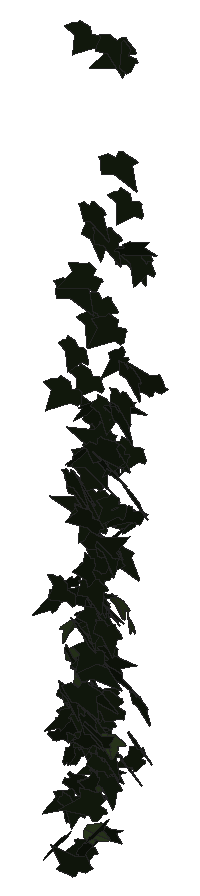
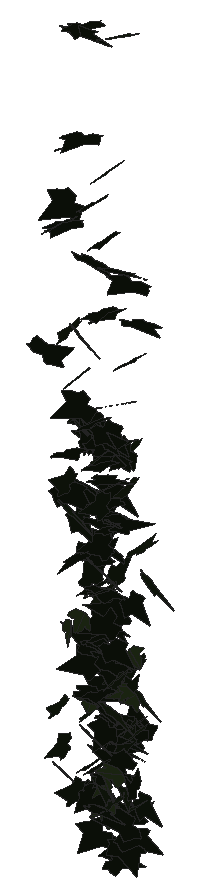
# SketchUp Ruby script. Lengths in inches.
U = 1.inch
M = Sketchup.active_model
def pt(a) = Geom::Point3d.new(a.map { |v| v * U })
def face(e, loops, mat)
  f = e.add_face(loops[0].map { |a| pt(a) })
  loops[1..].each { |l| e.add_face(l.map { |a| pt(a) }).erase! }
  f.material = f.back_material = mat if mat
  f
end
# faces: each face lists its corners as indices into pts; further lists are holes
def faces(e, pts, list, mat = nil) = list.each { |f| face(e, (f[0].is_a?(Array) ? f : [f]).map { |l| l.map { |i| pts[i] } }, mat) }
# xy, xz, yz: faces in a plane at the given z, y or x. An outline is a flat list of corners, or four numbers for a rectangle; further outlines are holes
def ring(l) = l.size == 4 ? [[l[0], l[1]], [l[2], l[1]], [l[2], l[3]], [l[0], l[3]]] : l.each_slice(2).to_a
def flat(e, list, mat, &to3) = list.each { |f| face(e, (f[0].is_a?(Array) ? f : [f]).map { |l| ring(l).map { |u, v| to3.(u, v) } }, mat) }
def xy(e, z, list, mat = nil) = flat(e, list, mat) { |x, y| [x, y, z] }
def xz(e, y, list, mat = nil) = flat(e, list, mat) { |x, z| [x, y, z] }
def yz(e, x, list, mat = nil) = flat(e, list, mat) { |y, z| [x, y, z] }
def lines(e, pts, list) = list.each { |a, b| e.add_line(pt(pts[a]), pt(pts[b])) }
# prism: a flat outline (further loops are holes) pulled along v
def prism(e, loops, v, mat = nil)
  f = face(e, loops, mat); d = Geom::Vector3d.new(v.map { |x| x * U })
  f.pushpull(f.normal.samedirection?(d) ? d.length : -d.length)
end
def box(e, o, s, mat = nil) = prism(e, [[o, [o[0] + s[0], o[1], o[2]], [o[0] + s[0], o[1] + s[1], o[2]], [o[0], o[1] + s[1], o[2]]]], [0, 0, s[2]], mat)
def at(x, y, z, deg = 0) = Geom::Transformation.translation(pt([x, y, z])) * Geom::Transformation.rotation(ORIGIN, Z_AXIS, deg.degrees)
def axes(o, x, y, z) = Geom::Transformation.new([*x, 0, *y, 0, *z, 0, *pt(o).to_a, 1])
def part(name) = M.definitions.add(name)
# library, detail: a bought-in or finely detailed component or shape, given as its bounding box
def library(name, o, s) = part(name).tap { |d| box(d.entities, o, s) }
def detail(e, o, s) = box(e.add_group.entities, o, s)
def put(e, d, t, mat = nil) = e.add_instance(d, t).tap { |i| i.material = mat if mat }
def group(e, t, mat = nil) = e.add_group.tap { |g| g.transformation = t; g.material = mat if mat }.entities
root = M.entities
M.materials.add("1026 AP 7946 SUNNY SIDE UP").color = [254, 231, 186]
M.materials.add("efeu1").color = [18, 25, 13]
M.materials.add("efeu2").color = [43, 57, 29]
c1 = part("ivyleaf_9")
p = [[1.54,2.16,1.25],[1.36,2.04,1.19],[-0.21,0.99,0.68],[-0.71,1.11,0.82],[-0.85,0.86,0.67],[-0.8,0.17,0.21],
  [-0.9,-0.01,0.1],[-0.67,-0.16,-0.02],[-0.08,-0.08,-0.05],[-0.03,-0.6,-0.4],[0.65,-0.88,-0.66],[0.83,-0.6,-0.49],
  [1.29,-0.42,-0.43],[1.8125,-0.07,-0.26],[1.21,0.44,0.15]]
faces(c1.entities,p,[[0,1,2,3,4,5,6,7,8,9,10,11,12,13,14]],"efeu1")
c2 = part("ivyleaf_10")
p = [[0,0.5,-0.03],[-0.0625,2.02,-0.43],[-0.19,2.01,-0.46],[-0.54,1.05,-0.29],[-0.52,0.625,-0.18],[-0.83,0.76,-0.28],
  [-1.16,0.64,-0.33],[-1.15,0.33,-0.24],[-0.77,-0.39,0.02],[-0.3,-0.51,0.16],[0.04,-0.48,0.23],[-0.02,2.01,-0.4375],
  [-0.06,2.01,-0.43],[0.04,-0.49,0.23],[0.67,-0.49,0.14],[1.38,0.36,-0.2],[1.375,0.51,-0.24],[0.81,0.65,-0.19],
  [0.62,0.59,-0.15],[0.6,1.09,-0.28],[0.5,1.23,-0.31]]
faces(c2.entities,p,[[0,1,2,3,4,5,6,7,8,9,10],[11,12,0,13,14,15,16,17,18,19,20]],"efeu2")
put(root,c1,axes([155.26,210.87,292.87],[-0.01471,0.06363,-0.46658],[-0.07177,-0.45123,-0.06693],[-0.71612,0.04391,0.01629]),"1026 AP 7946 SUNNY SIDE UP")
put(root,c2,axes([154.8125,211.34,299.78],[-0.45165,0.11821,-0.26149],[0.28889,-0.19606,-0.30858],[-0.33351,-0.3299,0.08683]),"1026 AP 7946 SUNNY SIDE UP")
put(root,c1,axes([154.84,211.07,297.82],[0.02248,-0.36054,0.12398],[0.01701,-0.12205,-0.37238],[0.59844,0.01701,0.00593]),"1026 AP 7946 SUNNY SIDE UP")
put(root,c2,axes([155.06,210.95,301.47],[-0.00156,-0.36293,0.18051],[0.07035,-0.17629,-0.37257],[0.63121,0.01875,0.04197]),"1026 AP 7946 SUNNY SIDE UP")
put(root,c1,axes([155.26,210.81,303.86],[-0.15823,0.26548,-0.30672],[0.14784,-0.28422,-0.29401],[-0.61139,-0.13744,0.00829]),"1026 AP 7946 SUNNY SIDE UP")
put(root,c1,axes([154.92,212.25,300.84],[0.02504,-0.38172,0.12372],[-0.01505,-0.12268,-0.39404],[0.63007,0.01224,-0.01433]),"1026 AP 7946 SUNNY SIDE UP")
put(root,c1,axes([155.13,212.25,330.74],[-0.4671,-0.33006,0.1928],[0.02957,-0.2523,-0.42487],[0.59734,-0.24561,0.1718]),"1026 AP 7946 SUNNY SIDE UP")
put(root,c1,axes([155.04,211.42,315.23],[-0.19853,-0.37754,0.19429],[-0.04235,-0.19148,-0.40993],[0.66376,-0.12514,0.03196]),"1026 AP 7946 SUNNY SIDE UP")
put(root,c1,axes([155.22,212.17,313.53],[-0.40682,-0.32312,0.1591],[0.03396,-0.2063,-0.40382],[0.56335,-0.2209,0.13924]),"1026 AP 7946 SUNNY SIDE UP")
put(root,c1,axes([155.63,211.75,299.06],[-0.29358,0.31866,0.1042],[-0.18846,0.04223,-0.37137],[-0.48983,-0.20723,0.08043]),"1026 AP 7946 SUNNY SIDE UP")
put(root,c1,axes([155.22,210.57,294.93],[-0.0047,-0.13169,0.44251],[0.32116,0.38302,0.12446],[-0.63047,0.19609,0.0601]),"1026 AP 7946 SUNNY SIDE UP")
put(root,c1,axes([155.74,211.33,307.43],[-0.25042,0.016,0.41643],[-0.63158,-0.05717,-0.16106],[0.07455,-0.4306,0.03429]),"1026 AP 7946 SUNNY SIDE UP")
put(root,c1,axes([155.46,210.92,292.41],[0.22088,0.28601,-0.25578],[-0.1803,-0.22209,-0.32954],[-0.56935,0.18129,0.00512]),"1026 AP 7946 SUNNY SIDE UP")
put(root,c1,axes([155.62,210.94,295.0625],[-0.09138,0.3352,0.31946],[-0.07881,0.3041,-0.34869],[-0.71165,-0.07672,-0.00241]),"1026 AP 7946 SUNNY SIDE UP")
put(root,c2,axes([154.95,212.11,296.42],[-0.23195,0.0092,-0.35759],[0.52484,-0.10038,-0.14944],[-0.15076,-0.3636,0.02991]),"1026 AP 7946 SUNNY SIDE UP")
put(root,c1,axes([155.5625,211.66,301.99],[-0.1227,0.24389,-0.30694],[0.01648,-0.30393,-0.25971],[-0.6069,-0.05757,0.055]),"1026 AP 7946 SUNNY SIDE UP")
put(root,c1,axes([155.6,212.07,312.29],[-0.09616,0.29316,-0.30507],[-0.03305,-0.30274,-0.30435],[-0.65624,-0.02771,0.06003]),"1026 AP 7946 SUNNY SIDE UP")
put(root,c1,axes([155.8,211.94,311.65],[0.00044,0.0373,0.46568],[-0.45064,0.3501,-0.02755],[-0.55235,-0.28561,0.02285]),"1026 AP 7946 SUNNY SIDE UP")
put(root,c1,axes([155.1,211.09,299.73],[0.04323,-0.27006,0.34706],[0.08101,-0.33466,-0.28138],[0.67597,0.05738,0.01153]),"1026 AP 7946 SUNNY SIDE UP")
put(root,c1,axes([155.41,211.02,297.08],[0.38899,-0.33905,-0.05305],[0.08149,-0.02341,0.43129],[-0.53259,-0.25121,0.02725]),"1026 AP 7946 SUNNY SIDE UP")
put(root,c1,axes([155.24,211.99,294.84],[0.07052,-0.36873,0.133],[0.06015,-0.12729,-0.38277],[0.61245,0.05496,0.02228]),"1026 AP 7946 SUNNY SIDE UP")
put(root,c1,axes([155.83,209.11,303.91],[-0.58678,0.26844,-0.11645],[0.11267,-0.09601,-0.47276],[-0.44488,-0.37837,0.03387]),"1026 AP 7946 SUNNY SIDE UP")
put(root,c1,axes([155.83,211.06,297.28],[-0.61329,-0.0879,0.09837],[-0.12809,-0.07162,-0.40901],[0.15961,-0.39523,0.04974]),"1026 AP 7946 SUNNY SIDE UP")
put(root,c1,axes([155.19,210.9,318.76],[-0.16822,-0.27026,-0.37246],[0.38117,0.27722,-0.28698],[0.59644,-0.25339,0.07835]),"1026 AP 7946 SUNNY SIDE UP")
put(root,c1,axes([155.93,211.31,319.24],[-0.66502,-0.08962,0.13802],[-0.14635,-0.17293,-0.42127],[0.20774,-0.40872,0.14505]),"1026 AP 7946 SUNNY SIDE UP")
put(root,c1,axes([155.0625,211.11,293.59],[0.17888,0.045,-0.43],[0.55093,0.22853,0.12502],[0.36437,-0.36763,0.02207]),"1026 AP 7946 SUNNY SIDE UP")
put(root,c1,axes([156.07,211.98,309.71],[-0.48184,-0.11851,0.26298],[-0.32753,-0.15974,-0.33404],[0.29903,-0.36592,0.05788]),"1026 AP 7946 SUNNY SIDE UP")
put(root,c2,axes([155.94,211.6,295.6],[0.29717,-0.28691,-0.22043],[-0.18347,0.17742,-0.3529],[0.53042,0.22211,0.00144]),"1026 AP 7946 SUNNY SIDE UP")
put(root,c1,axes([155.75,210.34,310.41],[0.19129,0.31428,0.32266],[0.21372,0.28081,-0.345],[-0.66205,0.18146,-0.01814]),"1026 AP 7946 SUNNY SIDE UP")
put(root,c1,axes([155.5,210.58,308.88],[0.28992,-0.39046,0.00796],[-0.01877,-0.01663,-0.44456],[0.61387,0.1839,-0.01735]),"1026 AP 7946 SUNNY SIDE UP")
put(root,c1,axes([155.625,212.15,321.09],[-0.02298,-0.45976,0.02714],[-0.02665,-0.02841,-0.47376],[0.72386,-0.01564,-0.01658]),"1026 AP 7946 SUNNY SIDE UP")
put(root,c1,axes([155.51,211.53,295.93],[-0.07021,-0.36024,-0.29873],[0.24166,0.26112,-0.35958],[0.68369,-0.12929,0.09643]),"1026 AP 7946 SUNNY SIDE UP")
put(root,c1,axes([155.89,212.41,304.63],[-0.3328,-0.28779,0.20701],[-0.06726,-0.2136,-0.3599],[0.54929,-0.20052,0.08135]),"1026 AP 7946 SUNNY SIDE UP")
put(root,c1,axes([155.375,211.17,296.19],[0.07114,-0.00259,0.42267],[0.60891,-0.13615,-0.04567],[0.21322,0.38968,-0.01059]),"1026 AP 7946 SUNNY SIDE UP")
put(root,c1,axes([156.21,212.05,294.36],[-0.57284,-0.01836,0.09846],[-0.14716,-0.03688,-0.37464],[0.04254,-0.37485,0.02981]),"1026 AP 7946 SUNNY SIDE UP")
put(root,c1,axes([155.8,211.65,298.04],[0.56708,0.02864,-0.12841],[-0.19494,-0.01532,-0.37275],[-0.05042,0.38132,-0.00309]),"1026 AP 7946 SUNNY SIDE UP")
put(root,c1,axes([155.7,212.35,311],[0.07175,-0.4252,0.08671],[0.00366,-0.08682,-0.44101],[0.6823,0.04518,-0.00675]),"1026 AP 7946 SUNNY SIDE UP")
put(root,c1,axes([156.39,211.61,310.85],[-0.13659,0.04509,0.4633],[-0.68656,-0.12572,-0.07468],[0.18209,-0.44019,0.06597]),"1026 AP 7946 SUNNY SIDE UP")
put(root,c1,axes([155.93,211.42,309.14],[-0.26759,-0.31249,0.23379],[-0.06516,-0.23369,-0.36206],[0.60541,-0.16327,0.06437]),"1026 AP 7946 SUNNY SIDE UP")
put(root,c1,axes([155.82,210.3,297.41],[-0.12906,-0.41377,0.22237],[-0.03657,-0.21765,-0.43548],[0.73463,-0.08353,0.01739]),"1026 AP 7946 SUNNY SIDE UP")
put(root,c1,axes([155.58,212.11,308.72],[0.51901,-0.25811,0.06094],[0.05048,-0.05718,-0.43123],[0.41382,0.33069,-0.02383]),"1026 AP 7946 SUNNY SIDE UP")
put(root,c1,axes([155.83,211.29,307.28],[-0.17095,-0.41693,-0.06387],[0.05381,0.05263,-0.44311],[0.66007,-0.11227,0.01958]),"1026 AP 7946 SUNNY SIDE UP")
put(root,c1,axes([155.48,210.07,296.9],[0.3105,0.02513,0.40691],[0.61573,0.05059,-0.20478],[-0.08881,0.43856,0.00291]),"1026 AP 7946 SUNNY SIDE UP")
put(root,c2,axes([155.83,210.52,299.32],[0.02607,-0.06883,-0.39514],[0.29621,0.33704,-0.05201],[0.5357,-0.18301,0.04799]),"1026 AP 7946 SUNNY SIDE UP")
put(root,c1,axes([155.56,210.81,303.11],[0.23731,0.06943,0.4262],[0.64186,0.07517,-0.16613],[-0.14929,0.43354,-0.03677]),"1026 AP 7946 SUNNY SIDE UP")
put(root,c1,axes([155.9,212.1,317.625],[-0.14908,-0.43327,-0.03563],[0.01685,0.03054,-0.45672],[0.68294,-0.09534,0.00349]),"1026 AP 7946 SUNNY SIDE UP")
put(root,c1,axes([155.875,212.21,296.51],[0.02171,-0.37853,-0.01415],[-0.01026,0.01135,-0.3901],[0.5954,0.014,-0.00621]),"1026 AP 7946 SUNNY SIDE UP")
put(root,c1,axes([155.78,210.87,299.88],[0.37027,-0.33282,-0.04085],[-0.06254,0.01806,-0.4193],[0.52297,0.2378,-0.02122]),"1026 AP 7946 SUNNY SIDE UP")
put(root,c1,axes([155.91,209.44,296.75],[0.55189,0.22058,0.20788],[-0.31932,-0.04986,0.42238],[0.34317,-0.40115,0.05871]),"1026 AP 7946 SUNNY SIDE UP")
put(root,c1,axes([155.95,212.14,299.88],[-0.17982,-0.38618,-0.05596],[0.02955,0.04879,-0.41461],[0.61202,-0.11582,0.00358]),"1026 AP 7946 SUNNY SIDE UP")
put(root,c1,axes([156.01,212.05,310.44],[-0.24093,-0.38921,0.01469],[0.04434,-0.02873,-0.42941],[0.61093,-0.1514,0.03696]),"1026 AP 7946 SUNNY SIDE UP")
put(root,c1,axes([156.03,211.69,304.46],[-0.42908,-0.23504,-0.17952],[0.24418,0.08347,-0.36885],[0.38845,-0.31209,0.03356]),"1026 AP 7946 SUNNY SIDE UP")
put(root,c2,axes([156.34,211.07,293.85],[-0.56885,-0.14746,0.06974],[-0.07219,-0.06774,-0.40022],[0.24528,-0.36192,0.04396]),"1026 AP 7946 SUNNY SIDE UP")
put(root,c1,axes([156.51,208.86,298.21],[-0.49126,0.25592,-0.07369],[0.06141,-0.06725,-0.41553],[-0.41392,-0.31371,0.02582]),"1026 AP 7946 SUNNY SIDE UP")
put(root,c1,axes([156.08,209.84,293.3],[-0.0865,-0.37987,0.16974],[0.02185,-0.16997,-0.39478],[0.65207,-0.0447,0.03574]),"1026 AP 7946 SUNNY SIDE UP")
put(root,c1,axes([156.25,211.41,317],[-0.27661,-0.39235,0.1516],[-0.0499,-0.14908,-0.44274],[0.65825,-0.17618,0.03014]),"1026 AP 7946 SUNNY SIDE UP")
put(root,c1,axes([156.625,212.05,297.84],[-0.52012,0.1902,-0.00951],[-0.01108,-0.03288,-0.39189],[-0.29931,-0.3293,0.03105]),"1026 AP 7946 SUNNY SIDE UP")
put(root,c1,axes([156.55,211.13,294.9],[-0.04383,0.28083,0.2672],[-0.09204,0.25225,-0.28815],[-0.59229,-0.05998,0.025]),"1026 AP 7946 SUNNY SIDE UP")
put(root,c1,axes([156.52,210.3125,291.06],[-0.09752,-0.06728,-0.39748],[0.01254,-0.3904,0.06659],[-0.61512,0.00271,0.06438]),"1026 AP 7946 SUNNY SIDE UP")
put(root,c1,axes([155.85,211.34,302.84],[0.68965,-0.02656,0.13753],[0.20427,-0.05444,-0.45066],[0.06466,0.45527,-0.04316]),"1026 AP 7946 SUNNY SIDE UP")
put(root,c1,axes([156.09,211.04,308.1],[0.21738,-0.38565,-0.07102],[-0.04284,0.06113,-0.42166],[0.61391,0.14082,-0.00428]),"1026 AP 7946 SUNNY SIDE UP")
put(root,c1,axes([156.22,212.24,312.36],[-0.1663,-0.41779,0.06863],[-0.0051,-0.07031,-0.44416],[0.66581,-0.10489,0.01374]),"1026 AP 7946 SUNNY SIDE UP")
put(root,c1,axes([156.21,211.3,308.32],[-0.19615,-0.37877,-0.1423],[0.09799,0.12246,-0.4096],[0.62516,-0.13804,0.01955]),"1026 AP 7946 SUNNY SIDE UP")
put(root,c1,axes([156.48,211.5,307.4375],[-0.54891,-0.21692,-0.05477],[0.08678,0.00946,-0.4228],[0.33982,-0.3528,0.0195]),"1026 AP 7946 SUNNY SIDE UP")
put(root,c1,axes([156.97,210.54,298.08],[-0.36059,-0.06545,-0.37476],[-0.574,-0.02421,0.24167],[-0.0874,0.42903,-0.04096]),"1026 AP 7946 SUNNY SIDE UP")
put(root,c1,axes([156.1,211,310.43],[-0.27389,-0.24671,-0.38608],[0.50558,0.20968,-0.29604],[0.48943,-0.35465,0.08974]),"1026 AP 7946 SUNNY SIDE UP")
put(root,c1,axes([156.52,211.38,301.48],[-0.55627,-0.14727,-0.09875],[0.18527,-0.04139,-0.38608],[0.20401,-0.36396,0.08136]),"1026 AP 7946 SUNNY SIDE UP")
put(root,c1,axes([156.59,210.73,307.43],[-0.5648,-0.20268,-0.05101],[0.10531,-0.02102,-0.42176],[0.31026,-0.36183,0.05029]),"1026 AP 7946 SUNNY SIDE UP")
put(root,c1,axes([156.17,209.6,309.98],[0.34472,-0.41022,-0.01409],[-0.02912,0.00296,-0.4789],[0.64462,0.2195,-0.0141]),"1026 AP 7946 SUNNY SIDE UP")
put(root,c2,axes([156.48,211.12,294.87],[0.11043,0.3231,-0.19485],[-0.07853,-0.18451,-0.3416],[-0.5849,0.08578,0.00908]),"1026 AP 7946 SUNNY SIDE UP")
put(root,c1,axes([156.58,208.74,304.75],[-0.352,-0.21644,0.36608],[-0.06312,-0.39162,-0.27315],[0.65284,-0.15457,0.17097]),"1026 AP 7946 SUNNY SIDE UP")
put(root,c1,axes([156.18,211.24,306.3],[0.59068,-0.13229,0.10905],[0.13181,-0.08069,-0.40794],[0.23237,0.38206,-0.04579]),"1026 AP 7946 SUNNY SIDE UP")
put(root,c1,axes([157.09,209.83,308.06],[0.07764,0.03968,-0.42827],[-0.58806,-0.18256,-0.06475],[-0.29296,0.37698,0.01647]),"1026 AP 7946 SUNNY SIDE UP")
put(root,c1,axes([157.15,210.62,304.6],[-0.26763,0.28883,0.26241],[-0.2813,0.18532,-0.34074],[-0.53431,-0.24224,0.04795]),"1026 AP 7946 SUNNY SIDE UP")
put(root,c1,axes([156.39,210.76,302.42],[-0.01912,-0.02919,0.4872],[0.19287,-0.45732,-0.02849],[0.71991,0.12174,0.02057]),"1026 AP 7946 SUNNY SIDE UP")
put(root,c1,axes([156.65,209.68,291.1],[0.12418,0.12123,0.39643],[0.33128,0.32119,-0.14717],[-0.53981,0.225,0.00088]),"1026 AP 7946 SUNNY SIDE UP")
put(root,c1,axes([156.4375,209.03,299.42],[0.1931,-0.39014,0.19411],[0.07661,-0.18449,-0.42236],[0.67847,0.13187,-0.00755]),"1026 AP 7946 SUNNY SIDE UP")
put(root,c1,axes([156.99,208.4375,315.16],[-0.62892,-0.20938,0.03355],[-0.01804,-0.05059,-0.46361],[0.33299,-0.39819,0.03825]),"1026 AP 7946 SUNNY SIDE UP")
put(root,c1,axes([156.61,212.24,330.85],[-0.1757,-0.44881,-0.14194],[0.08793,0.12527,-0.47515],[0.73179,-0.12281,0.02301]),"1026 AP 7946 SUNNY SIDE UP")
put(root,c1,axes([157.22,212.14,330.44],[-0.71102,-0.06233,0.14022],[-0.20246,-0.06115,-0.46869],[0.12106,-0.46836,0.0397]),"1026 AP 7946 SUNNY SIDE UP")
put(root,c1,axes([156.7,209.96,297.54],[-0.43458,-0.32905,-0.19753],[0.22069,0.12976,-0.44136],[0.5551,-0.30919,0.02083]),"1026 AP 7946 SUNNY SIDE UP")
put(root,c1,axes([156.98,208.03,292.66],[-0.29928,0.25567,-0.29715],[0.2036,-0.26229,-0.32742],[-0.57267,-0.22687,0.03888]),"1026 AP 7946 SUNNY SIDE UP")
put(root,c1,axes([156.5625,210.92,303.625],[0.07361,-0.37327,0.22572],[0.13019,-0.21073,-0.38559],[0.66973,0.08199,0.05015]),"1026 AP 7946 SUNNY SIDE UP")
put(root,c1,axes([157.16,210.93,305.19],[0.23744,0.09667,0.42573],[-0.65971,-0.02826,0.16481],[0.09486,-0.43855,0.08052]),"1026 AP 7946 SUNNY SIDE UP")
put(root,c1,axes([156.6,210.44,323.28],[0.25002,-0.4415,-0.10511],[-0.00948,0.10341,-0.48192],[0.71157,0.1565,0.03051]),"1026 AP 7946 SUNNY SIDE UP")
put(root,c1,axes([156.75,211.21,294.55],[0.47756,0.22921,0.05541],[0.08629,0.01427,-0.39128],[-0.35953,0.30788,-0.02031]),"1026 AP 7946 SUNNY SIDE UP")
put(root,c1,axes([156.78,211.02,295.11],[-0.08075,-0.40435,0.03952],[-0.00071,-0.04092,-0.42012],[0.63901,-0.05114,0.00453]),"1026 AP 7946 SUNNY SIDE UP")
put(root,c2,axes([156.97,211.89,302.95],[-0.55397,0.17413,-0.0598],[0.0618,-0.05333,-0.40398],[-0.28242,-0.35322,0.0289]),"1026 AP 7946 SUNNY SIDE UP")
put(root,c1,axes([156.61,209.81,309.55],[0.18261,-0.24852,0.38174],[0.17556,-0.35602,-0.28305],[0.68114,0.15839,-0.02939]),"1026 AP 7946 SUNNY SIDE UP")
put(root,c1,axes([156.51,210.36,300.31],[0.06638,-0.20487,-0.43862],[0.48458,0.3346,-0.1328],[0.56099,-0.26479,0.16661]),"1026 AP 7946 SUNNY SIDE UP")
put(root,c1,axes([156.85,211.79,312.81],[0.52366,0.18423,0.21515],[0.29357,0.09166,-0.39144],[-0.32326,0.38169,-0.00696]),"1026 AP 7946 SUNNY SIDE UP")
put(root,c1,axes([157.37,209.72,301.5],[-0.62914,-0.07619,-0.09519],[0.15241,-0.01929,-0.41806],[0.10972,-0.4101,0.03486]),"1026 AP 7946 SUNNY SIDE UP")
put(root,c1,axes([157.18,210.2,303.03],[-0.51809,-0.1456,-0.22824],[0.34378,0.04832,-0.36879],[0.23384,-0.39363,0.0365]),"1026 AP 7946 SUNNY SIDE UP")
put(root,c1,axes([157,211.03,321.89],[0.11826,-0.44232,-0.09429],[0.02379,0.09266,-0.46064],[0.70904,0.07066,0.03118]),"1026 AP 7946 SUNNY SIDE UP")
put(root,c1,axes([157.35,210.73,301.27],[-0.35812,-0.29538,0.17106],[-0.10226,-0.16028,-0.38271],[0.52423,-0.23305,0.0422]),"1026 AP 7946 SUNNY SIDE UP")
put(root,c1,axes([156.98,211.75,325.3125],[-0.04713,-0.35712,-0.31922],[0.16443,0.29574,-0.3622],[0.7229,-0.09055,0.06158]),"1026 AP 7946 SUNNY SIDE UP")
put(root,c1,axes([156.98,212.17,294.875],[0.39022,-0.30982,0.13998],[0.10225,-0.12391,-0.40884],[0.52317,0.2553,-0.0245]),"1026 AP 7946 SUNNY SIDE UP")
put(root,c1,axes([157.91,210.5625,298.54],[-0.25238,-0.20731,-0.37431],[-0.39098,-0.26411,0.26773],[-0.52696,0.29524,-0.01937]),"1026 AP 7946 SUNNY SIDE UP")
put(root,c1,axes([157.12,209.01,299.83],[-0.19995,-0.26152,-0.35993],[0.29912,0.29258,-0.29651],[0.61551,-0.22714,0.02717]),"1026 AP 7946 SUNNY SIDE UP")
put(root,c1,axes([157.26,210.25,292.1],[0.48179,0.2637,0.09544],[0.14089,0.0352,-0.41503],[-0.41547,0.31773,-0.03007]),"1026 AP 7946 SUNNY SIDE UP")
put(root,c1,axes([157.68,211.3,315.71],[-0.60953,0.15558,-0.16435],[0.21055,-0.09544,-0.42925],[-0.28132,-0.40852,0.03483]),"1026 AP 7946 SUNNY SIDE UP")
put(root,c1,axes([157.16,211.75,312.49],[0.24647,-0.40054,0.07353],[0.01137,-0.07616,-0.44304],[0.64027,0.15554,-0.02043]),"1026 AP 7946 SUNNY SIDE UP")
put(root,c1,axes([157.48,212.29,310.625],[-0.34619,-0.35384,0.05655],[-0.01766,-0.05994,-0.42909],[0.56325,-0.21936,0.02131]),"1026 AP 7946 SUNNY SIDE UP")
put(root,c1,axes([157.29,211.58,305.57],[0.17022,-0.31928,-0.27301],[-0.04857,0.26505,-0.34279],[0.64881,0.10361,0.04596]),"1026 AP 7946 SUNNY SIDE UP")
put(root,c1,axes([157.3,211.16,310.39],[-0.09882,0.07776,0.4577],[0.10959,-0.44107,0.0872],[0.7,0.08003,0.05096]),"1026 AP 7946 SUNNY SIDE UP")
put(root,c1,axes([157.0625,210.46,311.45],[0.01061,-0.13911,-0.4408],[0.53903,0.27761,-0.08594],[0.45639,-0.32464,0.11175]),"1026 AP 7946 SUNNY SIDE UP")
put(root,c1,axes([157.77,211.19,307.09],[-0.26053,0.34686,-0.2191],[0.12222,-0.20059,-0.39691],[-0.62964,-0.18246,0.01361]),"1026 AP 7946 SUNNY SIDE UP")
put(root,c2,axes([157.7,211.81,302.26],[-0.37502,0.28087,0.15348],[-0.20473,0.08146,-0.3765],[-0.4548,-0.26827,0.04293]),"1026 AP 7946 SUNNY SIDE UP")
put(root,c1,axes([157.73,210.89,308.47],[-0.63545,-0.03433,-0.1037],[0.1652,-0.07248,-0.4103],[0.02401,-0.41007,0.07871]),"1026 AP 7946 SUNNY SIDE UP")
put(root,c1,axes([157.91,207.8,291.53],[0.17034,0.06525,0.41415],[-0.63788,0.04973,0.10469],[-0.04989,-0.41301,0.07552]),"1026 AP 7946 SUNNY SIDE UP")
put(root,c1,axes([157.08,210.51,310.61],[0.41586,-0.24173,0.25625],[0.25848,-0.19004,-0.3694],[0.48201,0.31047,-0.02299]),"1026 AP 7946 SUNNY SIDE UP")
put(root,c1,axes([158.1,211.5,307.55],[-0.46386,0.30276,0.04876],[-0.09249,0.00612,-0.43371],[-0.47246,-0.29844,0.03703]),"1026 AP 7946 SUNNY SIDE UP")
put(root,c1,axes([157.22,209.69,299.47],[0.08581,-0.01498,-0.41708],[0.60102,0.13705,0.04866],[0.21074,-0.38475,0.03104]),"1026 AP 7946 SUNNY SIDE UP")
put(root,c1,axes([157.78,209.24,295],[-0.05,0.01914,0.40495],[-0.32138,-0.33769,-0.00207],[0.52862,-0.20349,0.03704]),"1026 AP 7946 SUNNY SIDE UP")
put(root,c1,axes([157.4375,209.5,304.97],[-0.28653,-0.17251,-0.34229],[0.54874,0.05272,-0.22574],[0.2093,-0.3744,0.12324]),"1026 AP 7946 SUNNY SIDE UP")
put(root,c1,axes([157.53,211.4,313.71],[0.12798,-0.42637,0.02202],[-0.00868,-0.02527,-0.4472],[0.67141,0.08095,-0.00998]),"1026 AP 7946 SUNNY SIDE UP")
put(root,c2,axes([157.57,209.19,292.69],[0.10106,0.19412,0.34889],[0.19888,0.31318,-0.20851],[-0.5791,0.14143,-0.01072]),"1026 AP 7946 SUNNY SIDE UP")
put(root,c1,axes([157.37,210.7,300.12],[0.65065,-0.15765,0.14147],[0.17728,-0.09052,-0.4546],[0.27794,0.42677,-0.04121]),"1026 AP 7946 SUNNY SIDE UP")
put(root,c1,axes([157.96,208.5,302.85],[0.28039,-0.40433,0.11874],[-0.03917,0.11731,0.45528],[-0.66094,-0.17848,0.02339]),"1026 AP 7946 SUNNY SIDE UP")
put(root,c1,axes([158.25,211.81,295.48],[-0.54445,0.20621,0.02357],[-0.05541,-0.01689,-0.41392],[-0.3213,-0.34652,0.03145]),"1026 AP 7946 SUNNY SIDE UP")
put(root,c1,axes([157.98,208.75,306.18],[-0.10167,-0.08351,0.45944],[-0.30484,-0.40273,-0.10889],[0.64584,-0.20324,0.02093]),"1026 AP 7946 SUNNY SIDE UP")
put(root,c1,axes([158.11,210.8,311.17],[-0.58365,0.09413,-0.18934],[0.24362,-0.12458,-0.38769],[-0.21578,-0.39526,0.07443]),"1026 AP 7946 SUNNY SIDE UP")
put(root,c1,axes([157.4,210.45,300.76],[0.13398,-0.0594,0.44769],[0.5672,-0.24295,-0.10841],[0.39326,0.37064,0.00384]),"1026 AP 7946 SUNNY SIDE UP")
put(root,c1,axes([157.77,209.09,292.51],[0.19666,0.3827,0.18178],[-0.11679,-0.15886,0.41336],[0.65082,-0.14415,0.01925]),"1026 AP 7946 SUNNY SIDE UP")
put(root,c1,axes([158.28,211.24,308.18],[-0.00642,0.19203,-0.40746],[-0.13034,-0.38988,-0.19588],[-0.68051,0.07286,0.04136]),"1026 AP 7946 SUNNY SIDE UP")
put(root,c1,axes([157.85,210.11,295.03],[0.01599,-0.42933,0.03587],[-0.00074,-0.03728,-0.44264],[0.67762,0.01009,-0.00133]),"1026 AP 7946 SUNNY SIDE UP")
put(root,c1,axes([157.83,208.59,298.72],[0.37903,-0.37115,-0.14351],[-0.147,0.10268,-0.45478],[0.60458,0.25765,-0.02061]),"1026 AP 7946 SUNNY SIDE UP")
put(root,c1,axes([157.82,210.14,303.55],[-0.07401,-0.19719,0.4071],[0.21423,-0.38563,-0.18326],[0.66221,0.10271,0.10479]),"1026 AP 7946 SUNNY SIDE UP")
put(root,c1,axes([157.92,211.78,320.91],[-0.09451,-0.4154,-0.19842],[0.12634,0.17928,-0.42839],[0.70722,-0.08754,0.05001]),"1026 AP 7946 SUNNY SIDE UP")
put(root,c1,axes([157.78,209.51,306.88],[-0.13674,-0.0105,0.47022],[0.71475,-0.04602,0.08785],[0.06802,0.46242,0.02216]),"1026 AP 7946 SUNNY SIDE UP")
put(root,c1,axes([158.24,208.58,297.61],[0.49702,0.10542,0.32396],[-0.49483,-0.0392,0.33984],[0.1618,-0.44372,0.04418]),"1026 AP 7946 SUNNY SIDE UP")
put(root,c1,axes([157.8,211.7,308.78],[0.32625,-0.32827,0.18789],[0.12891,-0.16592,-0.40063],[0.57771,0.22241,-0.01671]),"1026 AP 7946 SUNNY SIDE UP")
put(root,c1,axes([157.97,209.99,306.92],[0.0625,-0.44135,0.14165],[0.02486,-0.13914,-0.45731],[0.72763,0.04266,0.00346]),"1026 AP 7946 SUNNY SIDE UP")
put(root,c1,axes([158.53,209.75,318.23],[-0.73122,-0.05996,-0.02634],[0.04828,-0.04177,-0.48103],[0.09017,-0.46384,0.04394]),"1026 AP 7946 SUNNY SIDE UP")
put(root,c1,axes([158.77,208.22,294.875],[-0.65147,0.03325,0.20049],[-0.30895,-0.0297,-0.42628],[-0.02734,-0.4567,0.03962]),"1026 AP 7946 SUNNY SIDE UP")
put(root,c1,axes([157.99,211.61,296.52],[0.49504,-0.25897,-0.03859],[-0.06968,0.00266,-0.4191],[0.40517,0.31687,-0.02493]),"1026 AP 7946 SUNNY SIDE UP")
put(root,c1,axes([158.14,209.72,302.96],[-0.02097,-0.41757,-0.0092],[0.00099,0.00654,-0.43036],[0.65667,-0.01334,0.00036]),"1026 AP 7946 SUNNY SIDE UP")
put(root,c1,axes([158.0625,211.91,298.36],[0.21938,-0.34368,0.10329],[0.04886,-0.09768,-0.38261],[0.56167,0.14273,-0.00706]),"1026 AP 7946 SUNNY SIDE UP")
put(root,c1,axes([158.09,211.08,321.5],[0.49292,0.25656,0.22675],[0.29881,0.1121,-0.41555],[-0.43778,0.36539,-0.02833]),"1026 AP 7946 SUNNY SIDE UP")
put(root,c1,axes([158.41,210.98,324.01],[-0.33573,-0.36508,0.19299],[-0.03026,-0.20431,-0.42923],[0.646,-0.1993,0.08019]),"1026 AP 7946 SUNNY SIDE UP")
put(root,c1,axes([158.36,211.84,320.65],[-0.20185,-0.41381,0.17033],[-0.03457,-0.16841,-0.44647],[0.70122,-0.12742,0.02702]),"1026 AP 7946 SUNNY SIDE UP")
put(root,c1,axes([158.28,209.46,297.07],[0.18761,-0.42849,-0.0078],[-0.01779,0.00218,-0.45809],[0.67358,0.11941,-0.00993]),"1026 AP 7946 SUNNY SIDE UP")
put(root,c2,axes([158.35,209.45,297.52],[0.55419,0.15626,0.09655],[0.16161,-0.0043,-0.39456],[-0.23571,0.36444,-0.04353]),"1026 AP 7946 SUNNY SIDE UP")
put(root,c1,axes([159.03,211.76,314.42],[0.099,-0.00207,0.45436],[-0.59233,0.23148,0.05787],[-0.36072,-0.38067,0.02967]),"1026 AP 7946 SUNNY SIDE UP")
put(root,c1,axes([158.27,211.02,315.41],[0.1966,-0.42691,0.12957],[0.03831,-0.1264,-0.45886],[0.69984,0.12685,-0.01128]),"1026 AP 7946 SUNNY SIDE UP")
